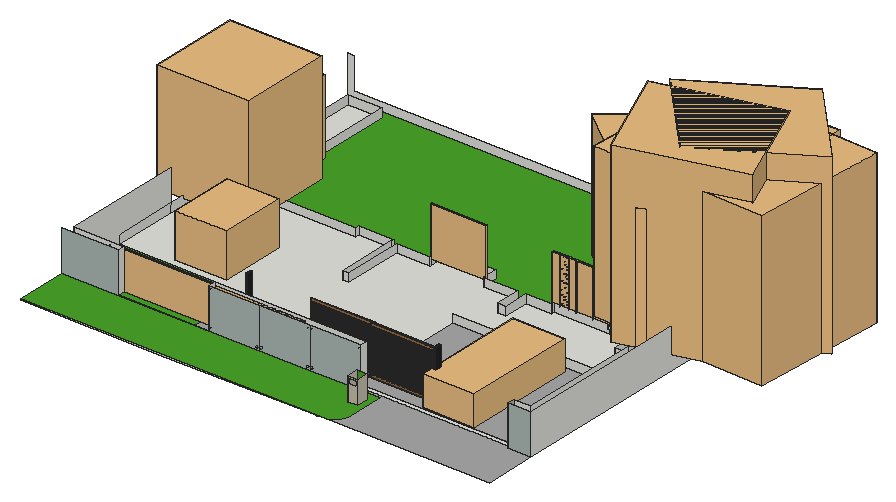
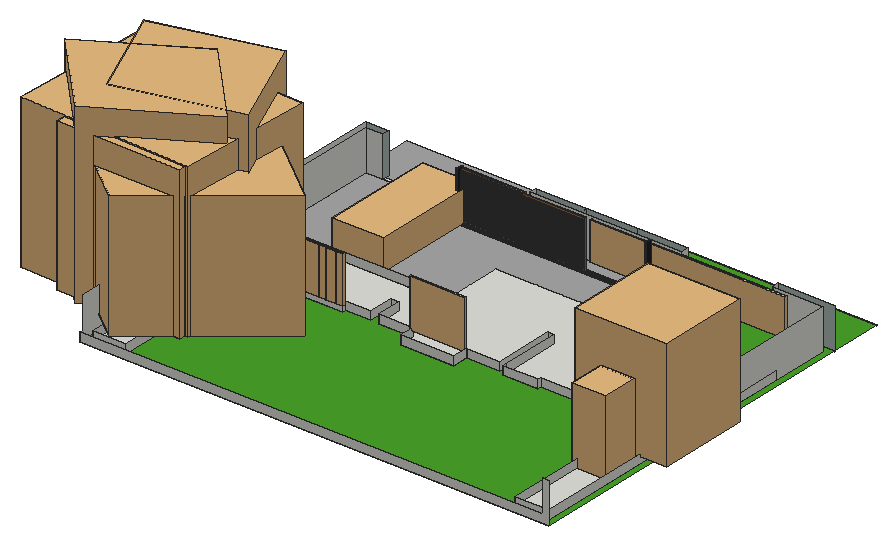
# SketchUp Ruby script. Lengths in inches.
U = 1.inch
M = Sketchup.active_model
def pt(a) = Geom::Point3d.new(a.map { |v| v * U })
def face(e, loops, mat)
  f = e.add_face(loops[0].map { |a| pt(a) })
  loops[1..].each { |l| e.add_face(l.map { |a| pt(a) }).erase! }
  f.material = f.back_material = mat if mat
  f
end
# faces: each face lists its corners as indices into pts; further lists are holes
def faces(e, pts, list, mat = nil) = list.each { |f| face(e, (f[0].is_a?(Array) ? f : [f]).map { |l| l.map { |i| pts[i] } }, mat) }
# xy, xz, yz: faces in a plane at the given z, y or x. An outline is a flat list of corners, or four numbers for a rectangle; further outlines are holes
def ring(l) = l.size == 4 ? [[l[0], l[1]], [l[2], l[1]], [l[2], l[3]], [l[0], l[3]]] : l.each_slice(2).to_a
def flat(e, list, mat, &to3) = list.each { |f| face(e, (f[0].is_a?(Array) ? f : [f]).map { |l| ring(l).map { |u, v| to3.(u, v) } }, mat) }
def xy(e, z, list, mat = nil) = flat(e, list, mat) { |x, y| [x, y, z] }
def xz(e, y, list, mat = nil) = flat(e, list, mat) { |x, z| [x, y, z] }
def yz(e, x, list, mat = nil) = flat(e, list, mat) { |y, z| [x, y, z] }
def lines(e, pts, list) = list.each { |a, b| e.add_line(pt(pts[a]), pt(pts[b])) }
# prism: a flat outline (further loops are holes) pulled along v
def prism(e, loops, v, mat = nil)
  f = face(e, loops, mat); d = Geom::Vector3d.new(v.map { |x| x * U })
  f.pushpull(f.normal.samedirection?(d) ? d.length : -d.length)
end
def box(e, o, s, mat = nil) = prism(e, [[o, [o[0] + s[0], o[1], o[2]], [o[0] + s[0], o[1] + s[1], o[2]], [o[0], o[1] + s[1], o[2]]]], [0, 0, s[2]], mat)
def at(x, y, z, deg = 0) = Geom::Transformation.translation(pt([x, y, z])) * Geom::Transformation.rotation(ORIGIN, Z_AXIS, deg.degrees)
def axes(o, x, y, z) = Geom::Transformation.new([*x, 0, *y, 0, *z, 0, *pt(o).to_a, 1])
def part(name) = M.definitions.add(name)
# library, detail: a bought-in or finely detailed component or shape, given as its bounding box
def library(name, o, s) = part(name).tap { |d| box(d.entities, o, s) }
def detail(e, o, s) = box(e.add_group.entities, o, s)
def put(e, d, t, mat = nil) = e.add_instance(d, t).tap { |i| i.material = mat if mat }
def group(e, t, mat = nil) = e.add_group.tap { |g| g.transformation = t; g.material = mat if mat }.entities
root = M.entities
M.materials.add("Material~3").color = [123, 113, 102]
M.materials.add("[0116_Lavender]").color = [73, 163, 41]
M.materials.add("[0132_LightGray]").color = [169, 169, 169]
M.materials.add("[0136_Charcoal]").color = [35, 35, 35]
M.materials.add("[Slate]").color = [172, 186, 182]
M.materials.add("[Tile Canvas]").color = [199, 192, 173]
M.materials.add("[Tile Grey]").color = [168, 168, 168]
M.materials.add("[Wood Floor Light]").color = [204, 176, 127]
M.materials.add("[Wood Floor]").color = [155, 105, 61]
c1 = library("Floor plant",[-5.56,-16.3125,0.81],[76.88,76.71,92.33])
c2 = library("Potted broadleaf plant",[-29.7,0,-10.87],[31.67,38.52,72.45])
c3 = library("Sem+nome (1)",[20.77,3.52,-2.22],[96.42,122.82,82.56])
c4 = library("Sliding Gate",[0,0,0],[194.88,4.13,70.58])
c5 = part("Group\#106")
box(c5.entities,[0,0,0],[3.9375,10.43,92.32])
c6 = library("3 door",[0,0,0],[74.8,3.9375,43.31])
c7 = part("Group\#107")
prism(c7.entities,[[[357.51,0,0.79],[357.51,0,-1.18],[357.51,10.43,-1.18],[357.51,10.43,0.79],[357.51,10.12,0.79],[357.51,10.12,0.39],[357.51,7.09,0.39],[357.51,7.09,0.79],[357.51,6.73,0.79],[357.51,6.73,0.39],[357.51,3.7,0.39],[357.51,3.7,0.79],[357.51,3.35,0.79],[357.51,3.35,0.39],[357.51,0.31,0.39],[357.51,0.31,0.79]]],[-357.51,0,0])
c8 = part("Group\#98")
box(c8.entities,[0,0,0],[1.57,1.97,82.68])
c9 = part("Group\#108")
g1 = group(c9.entities,at(0,0,0),"[Wood Floor]")
put(g1,c8,at(43.7,15.53,3.9375))
put(g1,c8,at(68.9,15.53,3.9375))
put(g1,c8,at(109.84,15.53,3.9375))
put(g1,c8,at(103.54,15.53,3.9375))
put(g1,c8,at(56.3,15.53,3.9375))
put(g1,c8,at(78.35,15.53,3.9375))
put(g1,c8,at(72.05,15.53,3.9375))
put(g1,c8,at(31.1,15.53,3.9375))
put(g1,c8,at(87.8,15.53,3.9375))
put(g1,c8,at(46.85,15.53,3.9375))
put(g1,c8,at(59.45,15.53,3.9375))
g2 = group(g1,at(12.2,15.53,3.9375))
box(g2,[0,0,0],[1.57,1.97,82.68])
put(g1,c8,at(50,15.53,3.9375))
put(g1,c8,at(106.69,15.53,3.9375))
put(g1,c8,at(34.25,15.53,3.9375))
put(g1,c8,at(81.5,15.53,3.9375))
put(g1,c8,at(53.15,15.53,3.9375))
put(g1,c8,at(27.95,15.53,3.9375))
put(g1,c8,at(65.75,15.53,3.9375))
put(g1,c8,at(18.5,15.53,3.9375))
put(g1,c8,at(40.55,15.53,3.9375))
put(g1,c8,at(75.2,15.53,3.9375))
put(g1,c8,at(21.65,15.53,3.9375))
put(g1,c8,at(62.6,15.53,3.9375))
put(g1,c8,at(84.65,15.53,3.9375))
put(g1,c8,at(100.39,15.53,3.9375))
put(g1,c8,at(112.99,15.53,3.9375))
put(g1,c8,at(24.8,15.53,3.9375))
put(g1,c8,at(37.4,15.53,3.9375))
put(g1,c8,at(97.24,15.53,3.9375))
put(g1,c8,at(2.76,15.53,3.9375))
g3 = group(g1,at(5.91,15.53,3.9375))
box(g3,[0,0,0],[1.57,1.97,82.68])
put(g1,c8,at(94.09,15.53,3.9375))
put(g1,c8,at(15.35,15.53,3.9375))
put(g1,c8,at(9.06,15.53,3.9375))
put(g1,c8,at(90.94,15.53,3.9375))
g4 = group(c9.entities,at(0,14.54,0))
xy(g4,0,[[0,0,118.11,2.95]],"[Wood Floor]")
xy(g4,3.9375,[[2.76,0,115.35,2.95]],"[Wood Floor]")
xy(g4,30.51,[[2.76,0,115.35,0.98]],"[Wood Floor]")
xy(g4,31.5,[[2.76,0,115.35,0.98]],"[Wood Floor]")
xy(g4,42.19,[[1.12,0,1.91,0.79]],"[Wood Floor]")
xy(g4,42.49,[[116.24,2.17,117.03,2.95]],"[Wood Floor]")
xy(g4,46.92,[[1.12,0,1.91,0.79]],"[Wood Floor]")
xy(g4,47.22,[[116.24,2.17,117.03,2.95]],"[Wood Floor]")
xy(g4,58.07,[[2.76,0,115.35,0.98]],"[Wood Floor Light]")
xy(g4,59.06,[[2.76,0,115.35,0.98]],"[Wood Floor]")
xy(g4,86.61,[[2.76,0,115.35,2.95]],"[Wood Floor]")
xy(g4,90.55,[[0,0,118.11,2.95]],"[Wood Floor]")
xz(g4,0,[[2.76,30.51,115.35,31.5],[2.76,58.07,115.35,59.06]],"[Wood Floor Light]")
xz(g4,0,[[[0,0,118.11,90.55],[2.76,3.9375,115.35,86.61],[1.12,42.19,1.91,46.92]]],"[Wood Floor]")
xz(g4,0.79,[[1.12,42.19,1.91,46.92]],"[Wood Floor]")
xz(g4,0.98,[[2.76,30.51,115.35,31.5],[2.76,58.07,115.35,59.06]],"[Wood Floor]")
xz(g4,2.17,[[116.24,42.49,117.03,47.22]],"[Wood Floor]")
xz(g4,2.95,[[[0,0,118.11,90.55],[2.76,3.9375,115.35,86.61],[116.24,42.49,117.03,47.22]]],"[Wood Floor]")
yz(g4,0,[[0,0,2.95,90.55]],"[Wood Floor]")
yz(g4,1.12,[[0,42.19,0.79,46.92]],"[Wood Floor]")
yz(g4,1.91,[[0,42.19,0.79,46.92]],"[Wood Floor]")
yz(g4,2.76,[[0,3.9375,2.95,3.9375,2.95,86.61,0,86.61,0,59.06,0.98,59.06,0.98,58.07,0,58.07,0,31.5,0.98,31.5,0.98,30.51,0,30.51],[0,30.51,0.98,31.5],[0,58.07,0.98,59.06]],"[Wood Floor]")
yz(g4,115.35,[[0,3.9375,0,30.51,0.98,30.51,0.98,31.5,0,31.5,0,58.07,0.98,58.07,0.98,59.06,0,59.06,0,86.61,2.95,86.61,2.95,3.9375],[0,30.51,0.98,31.5],[0,58.07,0.98,59.06]],"[Wood Floor]")
yz(g4,116.24,[[2.17,42.49,2.95,47.22]],"[Wood Floor]")
yz(g4,117.03,[[2.17,42.49,2.95,47.22]],"[Wood Floor]")
yz(g4,118.11,[[0,0,2.95,90.55]],"[Wood Floor]")
p = [[5.91,2.95,86.61],[5.91,2.95,3.9375]]
lines(g4,p,[[0,1]])
c10 = part("Group\#103")
put(c10.entities,c8,at(43.7,15.53,3.9375))
put(c10.entities,c8,at(68.9,15.53,3.9375))
put(c10.entities,c8,at(109.84,15.53,3.9375))
put(c10.entities,c8,at(103.54,15.53,3.9375))
put(c10.entities,c8,at(56.3,15.53,3.9375))
put(c10.entities,c8,at(78.35,15.53,3.9375))
put(c10.entities,c8,at(72.05,15.53,3.9375))
put(c10.entities,c8,at(31.1,15.53,3.9375))
put(c10.entities,c8,at(87.8,15.53,3.9375))
put(c10.entities,c8,at(46.85,15.53,3.9375))
put(c10.entities,c8,at(59.45,15.53,3.9375))
put(c10.entities,c8,at(12.2,15.53,3.9375))
put(c10.entities,c8,at(50,15.53,3.9375))
put(c10.entities,c8,at(106.69,15.53,3.9375))
put(c10.entities,c8,at(34.25,15.53,3.9375))
put(c10.entities,c8,at(81.5,15.53,3.9375))
put(c10.entities,c8,at(53.15,15.53,3.9375))
put(c10.entities,c8,at(27.95,15.53,3.9375))
put(c10.entities,c8,at(65.75,15.53,3.9375))
put(c10.entities,c8,at(18.5,15.53,3.9375))
put(c10.entities,c8,at(40.55,15.53,3.9375))
put(c10.entities,c8,at(75.2,15.53,3.9375))
put(c10.entities,c8,at(21.65,15.53,3.9375))
put(c10.entities,c8,at(62.6,15.53,3.9375))
put(c10.entities,c8,at(84.65,15.53,3.9375))
put(c10.entities,c8,at(100.39,15.53,3.9375))
put(c10.entities,c8,at(112.99,15.53,3.9375))
put(c10.entities,c8,at(24.8,15.53,3.9375))
put(c10.entities,c8,at(37.4,15.53,3.9375))
put(c10.entities,c8,at(97.24,15.53,3.9375))
put(c10.entities,c8,at(2.76,15.53,3.9375))
put(c10.entities,c8,at(5.91,15.53,3.9375))
put(c10.entities,c8,at(94.09,15.53,3.9375))
put(c10.entities,c8,at(15.35,15.53,3.9375))
put(c10.entities,c8,at(9.06,15.53,3.9375))
put(c10.entities,c8,at(90.94,15.53,3.9375))
c11 = part("Group\#104")
put(c11.entities,c10,at(0,0,0),"[Wood Floor]")
g5 = group(c11.entities,at(0,14.54,0))
xy(g5,0,[[0,0,118.11,2.95]],"[Wood Floor]")
xy(g5,3.9375,[[2.76,0,115.35,2.95]],"[Wood Floor]")
xy(g5,30.51,[[2.76,0,115.35,0.98]],"[Wood Floor]")
xy(g5,31.5,[[2.76,0,115.35,0.98]],"[Wood Floor]")
xy(g5,42.07,[[116.14,2.17,116.92,2.95]],"[Wood Floor]")
xy(g5,42.125,[[1.06,0,1.84,0.79]],"[Wood Floor]")
xy(g5,46.8,[[116.14,2.17,116.92,2.95]],"[Wood Floor]")
xy(g5,46.85,[[1.06,0,1.84,0.79]],"[Wood Floor]")
xy(g5,58.07,[[2.76,0,115.35,0.98]],"[Wood Floor Light]")
xy(g5,59.06,[[2.76,0,115.35,0.98]],"[Wood Floor]")
xy(g5,86.61,[[2.76,0,115.35,2.95]],"[Wood Floor]")
xy(g5,90.55,[[0,0,118.11,2.95]],"[Wood Floor]")
xz(g5,0,[[2.76,30.51,115.35,31.5],[2.76,58.07,115.35,59.06]],"[Wood Floor Light]")
xz(g5,0,[[[0,0,118.11,90.55],[2.76,3.9375,115.35,86.61],[1.06,42.125,1.84,46.85]]],"[Wood Floor]")
xz(g5,0.79,[[1.06,42.125,1.84,46.85]],"[Wood Floor]")
xz(g5,0.98,[[2.76,30.51,115.35,31.5],[2.76,58.07,115.35,59.06]],"[Wood Floor]")
xz(g5,2.17,[[116.14,42.07,116.92,46.8]],"[Wood Floor]")
xz(g5,2.95,[[[0,0,118.11,90.55],[2.76,3.9375,115.35,86.61],[116.14,42.07,116.92,46.8]]],"[Wood Floor]")
yz(g5,0,[[0,0,2.95,90.55]],"[Wood Floor]")
yz(g5,1.06,[[0,42.125,0.79,46.85]],"[Wood Floor]")
yz(g5,1.84,[[0,42.125,0.79,46.85]],"[Wood Floor]")
yz(g5,2.76,[[0,3.9375,2.95,3.9375,2.95,86.61,0,86.61,0,59.06,0.98,59.06,0.98,58.07,0,58.07,0,31.5,0.98,31.5,0.98,30.51,0,30.51],[0,30.51,0.98,31.5],[0,58.07,0.98,59.06]],"[Wood Floor]")
yz(g5,115.35,[[0,3.9375,0,30.51,0.98,30.51,0.98,31.5,0,31.5,0,58.07,0.98,58.07,0.98,59.06,0,59.06,0,86.61,2.95,86.61,2.95,3.9375],[0,30.51,0.98,31.5],[0,58.07,0.98,59.06]],"[Wood Floor]")
yz(g5,116.14,[[2.17,42.07,2.95,46.8]],"[Wood Floor]")
yz(g5,116.92,[[2.17,42.07,2.95,46.8]],"[Wood Floor]")
yz(g5,118.11,[[0,0,2.95,90.55]],"[Wood Floor]")
p = [[5.91,2.95,86.61],[5.91,2.95,3.9375]]
lines(g5,p,[[0,1]])
c12 = library("3DGeom~4_Defintion",[362.52,-15.59,12.6],[288.85,70.11,1000])
c13 = library("BMW 8 Series M850i 2019",[-14.25,0.77,-0.16],[87.38,190.63,50.87])
c14 = library("Group\#65",[-33.32,-34.9375,32.67],[162.87,159.66,128.34])
c15 = library("Group\#81",[-10.45,-6.67,0],[121.7,116.61,164.95])
c16 = library("Group\#82",[-10.45,-6.67,0],[121.7,116.61,164.95])
c17 = library("Group\#69",[-10.45,-6.67,0],[121.7,116.61,164.95])
c18 = library("Group\#83",[-33.32,-34.9375,32.67],[162.87,159.66,128.34])
c19 = library("Group\#64",[-33.32,-34.9375,81.35],[162.87,159.66,79.66])
c20 = library("Group\#80",[-33.32,-34.9375,77.91],[162.87,159.66,83.1])
c21 = part("Palem Elek")
put(c21.entities,c14,axes([92.2,20.3,-29.73],[0.70711,0.70711,0],[-0.70711,0.70711,0],[0,0,0.91208]))
put(c21.entities,c15,axes([60.27,20.78,0],[1,0,0],[0,1,0],[0,0,0.85762]))
put(c21.entities,c16,at(25.45,60.83,0,-53.5))
put(c21.entities,c17,at(84.4375,135.48,0,-161.4))
put(c21.entities,c18,axes([38.54,105.7,-36.19],[-0.04013,-0.99919,0],[0.99919,-0.04013,0],[0,0,1.11001]))
put(c21.entities,c19,axes([57.15,96.51,-54.45],[-0.02003,-0.49872,0.02965],[0.4996,-0.02007,0],[0.00123,0.03065,0.51628]))
put(c21.entities,c20,axes([74.94,50.39,-54.06],[0.40095,0.29715,0.03075],[-0.29654,0.38966,0.10114],[0.04012,-0.11026,0.54246]))
c22 = part("palem elek\#1")
put(c22.entities,c21,at(-81.14,-74.56,-0.83))
c23 = part("Coqueiro")
put(c23.entities,c22,axes([83.17,89.39,9.5625],[0,1.1016,0],[-1.377,0,0],[0,0,1.39284]))
xy(root,-10.51,[[1716.62,498.28,1993.42,505.1],[[1168.49,611.53,1168.49,1146.63,1232.12,1146.63,1232.12,732.28,1243.06,732.28,1243.06,845.35,1425.1,845.35,1425.1,851.0625,1490.48,851.0625,1490.48,732.28,1501.42,732.28,1501.42,845.35,1564.1,845.35,1564.1,874.25,1664.38,874.25,1664.38,845.35,1728.67,845.35,1728.67,798.41,1744,798.41,1744,845.35,1791.45,845.35,1791.45,851.0625,1960.87,851.0625,1960.87,1146.63,2024.12,1146.63,2024.12,732.28,1696.41,732.28,1696.41,611.53],[1945.54,801.78,1960.87,845.35]]])
xy(root,-10.51,[[[1156.87,393.78,1727.12,393.78,1730.14,394.71,1733.08,395.9,1735.89,397.35,1738.57,399.04,1741.08,400.97,1743.42,403.1,1745.56,405.44,1747.48,407.96,1749.17,410.63,1750.62,413.45,1751.8125,416.38,1752.74,419.41,1752.74,491.47,1716.62,491.47,1716.62,505.1,1431.76,505.1,1431.76,491.47,1262.76,491.47,1262.76,505.1,1168.49,505.1,1168.49,1146.63,1232.12,1146.63,1232.12,732.28,1243.06,732.28,1243.06,845.35,1425.1,845.35,1425.1,851.0625,1490.48,851.0625,1490.48,732.28,1501.42,732.28,1501.42,845.35,1564.1,845.35,1564.1,874.25,1664.38,874.25,1664.38,845.35,1728.67,845.35,1728.67,798.41,1744,798.41,1744,845.35,1791.45,845.35,1791.45,851.0625,1960.87,851.0625,1960.87,1146.63,2024.12,1146.63,2024.12,505.1,1993.42,505.1,1993.42,491.47,2036.12,491.47,2036.12,1160.85,1156.87,1160.85],[1722.63,453.42,1741.07,475.99]],[1262.76,491.47,1406.2,491.47,1411.4,611.53,1168.49,611.53,1168.49,505.1,1262.76,505.1]],"[0116_Lavender]")
xy(root,-10.51,[[1727.12,393.78,2036.12,393.78,2036.12,491.47,1993.42,491.47,1993.42,498.28,1716.62,498.28,1716.62,491.47,1752.74,491.47,1752.74,419.41,1751.8125,416.38,1750.62,413.45,1749.17,410.63,1747.48,407.96,1745.56,405.44,1743.42,403.1,1741.08,400.97,1738.57,399.04,1735.89,397.35,1733.08,395.9,1730.14,394.71],[1406.2,491.47,1431.76,491.47,1431.76,505.1,2024.12,505.1,2024.12,732.28,1696.41,732.28,1696.41,611.53,1411.4,611.53]],"[Tile Grey]")
xz(root,393.78,[[1156.87,-12.6875,1431.76,-12.6875,1716.62,-10.51,1156.87,-10.51]])
xz(root,453.42,[[[1722.63,-10.51,1741.07,32.74],[1724.98,19.53,1739.11,29.34]]],"[Tile Canvas]")
xz(root,475.99,[[1722.63,-10.51,1741.07,32.74]],"[0116_Lavender]")
xz(root,491.47,[[1262.76,-12.6875,1431.76,-10.51]])
xz(root,491.47,[[1522.98,-7.89,1523.46,-7.82,1523.92,-7.63,1524.3,-7.34,1524.6,-6.95,1524.79,-6.5,1524.85,-6.01,1524.79,-5.52,1524.6,-5.07,1524.3,-4.68,1523.92,-4.39,1523.46,-4.2,1522.98,-4.14,1522.49,-4.2,1522.04,-4.39,1521.65,-4.68,1521.36,-5.07,1521.17,-5.52,1521.1,-6.01,1521.17,-6.5,1521.36,-6.95,1521.65,-7.34,1522.04,-7.63,1522.49,-7.82],[1617.93,-7.89,1618.41,-7.82,1618.87,-7.63,1619.26,-7.34,1619.55,-6.95,1619.74,-6.5,1619.8,-6.01,1619.74,-5.52,1619.55,-5.07,1619.26,-4.68,1618.87,-4.39,1618.41,-4.2,1617.93,-4.14,1617.44,-4.2,1616.99,-4.39,1616.6,-4.68,1616.31,-5.07,1616.12,-5.52,1616.05,-6.01,1616.12,-6.5,1616.31,-6.95,1616.6,-7.34,1616.99,-7.63,1617.44,-7.82],[1712.88,-7.89,1713.37,-7.82,1713.82,-7.63,1714.21,-7.34,1714.5,-6.95,1714.69,-6.5,1714.76,-6.01,1714.69,-5.52,1714.5,-5.07,1714.21,-4.68,1713.82,-4.39,1713.37,-4.2,1712.88,-4.14,1712.4,-4.2,1711.94,-4.39,1711.55,-4.68,1711.26,-5.07,1711.07,-5.52,1711.01,-6.01,1711.07,-6.5,1711.26,-6.95,1711.55,-7.34,1711.94,-7.63,1712.4,-7.82],[1435.25,-6.41,1435.73,-6.4,1436.2,-6.26,1436.62,-6.01,1436.96,-5.66,1437.19,-5.23,1437.31,-4.75,1437.3,-4.26,1437.16,-3.79,1436.9,-3.375,1436.55,-3.04,1436.12,-2.8,1435.65,-2.6875,1435.16,-2.7,1434.6875,-2.84,1434.27,-3.09,1433.93,-3.45,1433.7,-3.875,1433.58,-4.35,1433.59,-4.84,1433.73,-5.31,1433.99,-5.73,1434.34,-6.07,1434.77,-6.3],[1530.2,-6.41,1530.6875,-6.4,1531.16,-6.26,1531.57,-6.01,1531.91,-5.66,1532.15,-5.23,1532.26,-4.75,1532.25,-4.26,1532.11,-3.79,1531.86,-3.375,1531.5,-3.04,1531.07,-2.8,1530.6,-2.6875,1530.11,-2.7,1529.64,-2.84,1529.22,-3.09,1528.88,-3.45,1528.65,-3.875,1528.53,-4.35,1528.54,-4.84,1528.68,-5.31,1528.9375,-5.73,1529.29,-6.07,1529.72,-6.3],
  [1625.15,-6.41,1625.64,-6.4,1626.11,-6.26,1626.52,-6.01,1626.86,-5.66,1627.1,-5.23,1627.21,-4.75,1627.2,-4.26,1627.0625,-3.79,1626.81,-3.375,1626.45,-3.04,1626.02,-2.8,1625.55,-2.6875,1625.06,-2.7,1624.59,-2.84,1624.17,-3.09,1623.83,-3.45,1623.6,-3.875,1623.48,-4.35,1623.49,-4.84,1623.63,-5.31,1623.89,-5.73,1624.24,-6.07,1624.67,-6.3]],"[0132_LightGray]")
xz(root,491.47,[[1156.87,-12.6875,1262.76,65.1875],[[1431.76,-12.6875,1716.62,-10.51,1716.62,65.1875,1431.76,65.1875],[1522.98,-7.89,1522.49,-7.82,1522.04,-7.63,1521.65,-7.34,1521.36,-6.95,1521.17,-6.5,1521.1,-6.01,1521.17,-5.52,1521.36,-5.07,1521.65,-4.68,1522.04,-4.39,1522.49,-4.2,1522.98,-4.14,1523.46,-4.2,1523.92,-4.39,1524.3,-4.68,1524.6,-5.07,1524.79,-5.52,1524.85,-6.01,1524.79,-6.5,1524.6,-6.95,1524.3,-7.34,1523.92,-7.63,1523.46,-7.82],[1617.93,-7.89,1617.44,-7.82,1616.99,-7.63,1616.6,-7.34,1616.31,-6.95,1616.12,-6.5,1616.05,-6.01,1616.12,-5.52,1616.31,-5.07,1616.6,-4.68,1616.99,-4.39,1617.44,-4.2,1617.93,-4.14,1618.41,-4.2,1618.87,-4.39,1619.26,-4.68,1619.55,-5.07,1619.74,-5.52,1619.8,-6.01,1619.74,-6.5,1619.55,-6.95,1619.26,-7.34,1618.87,-7.63,1618.41,-7.82],[1522.98,57.74,1522.49,57.8,1522.04,57.99,1521.65,58.29,1521.36,58.68,1521.17,59.13,1521.1,59.61,1521.17,60.1,1521.36,60.55,1521.65,60.94,1522.04,61.24,1522.49,61.43,1522.98,61.49,1523.46,61.43,1523.92,61.24,1524.3,60.94,1524.6,60.55,1524.79,60.1,1524.85,59.61,1524.79,59.13,1524.6,58.68,1524.3,58.29,1523.92,57.99,1523.46,57.8],[1617.93,57.74,1617.44,57.8,1616.99,57.99,1616.6,58.29,1616.31,58.68,1616.12,59.13,1616.05,59.61,1616.12,60.1,1616.31,60.55,1616.6,60.94,1616.99,61.24,1617.44,61.43,1617.93,61.49,1618.41,61.43,1618.87,61.24,1619.26,60.94,1619.55,60.55,1619.74,60.1,1619.8,59.61,1619.74,59.13,1619.55,58.68,1619.26,58.29,1618.87,57.99,1618.41,57.8],[1712.88,-7.89,1712.4,-7.82,1711.94,-7.63,1711.55,-7.34,1711.26,-6.95,1711.07,-6.5,1711.01,-6.01,1711.07,-5.52,1711.26,-5.07,1711.55,-4.68,1711.94,-4.39,1712.4,-4.2,1712.88,-4.14,1713.37,-4.2,1713.82,-4.39,1714.21,-4.68,1714.5,-5.07,1714.69,-5.52,1714.76,-6.01,1714.69,-6.5,1714.5,-6.95,1714.21,-7.34,1713.82,-7.63,1713.37,-7.82],[1712.88,57.74,1712.4,57.8,1711.94,57.99,1711.55,58.29,1711.26,58.68,1711.07,59.13,1711.01,59.61,1711.07,60.1,1711.26,60.55,1711.55,60.94,1711.94,61.24,1712.4,61.43,1712.88,61.49,1713.37,61.43,1713.82,61.24,1714.21,60.94,1714.5,60.55,1714.69,60.1,1714.76,59.61,1714.69,59.13,1714.5,58.68,1714.21,58.29,1713.82,57.99,1713.37,57.8],[1530.2,59.21,1529.72,59.33,1529.29,59.56,1528.9375,59.9,1528.68,60.32,1528.54,60.78,1528.53,61.27,1528.65,61.75,1528.88,62.18,1529.22,62.53,1529.64,62.79,1530.11,62.93,1530.6,62.9375,1531.07,62.82,1531.5,62.59,1531.86,62.25,1532.11,61.83,1532.25,61.36,1532.26,60.875,1532.15,60.4,1531.91,59.97,1531.57,59.61,1531.16,59.36,1530.6875,59.22],[1625.15,59.21,1624.67,59.33,1624.24,59.56,1623.89,59.9,1623.63,60.32,1623.49,60.78,1623.48,61.27,1623.6,61.75,1623.83,62.18,1624.17,62.53,1624.59,62.79,1625.06,62.93,1625.55,62.9375,1626.02,62.82,1626.45,62.59,1626.81,62.25,1627.0625,61.83,1627.2,61.36,1627.21,60.875,1627.1,60.4,1626.86,59.97,1626.52,59.61,1626.11,59.36,1625.64,59.22],[1435.25,-6.41,1434.77,-6.3,1434.34,-6.07,1433.99,-5.73,1433.73,-5.31,1433.59,-4.84,1433.58,-4.35,1433.7,-3.875,1433.93,-3.45,1434.27,-3.09,1434.6875,-2.84,1435.16,-2.7,1435.65,-2.6875,1436.12,-2.8,1436.55,-3.04,1436.9,-3.375,1437.16,-3.79,1437.3,-4.26,1437.31,-4.75,1437.19,-5.23,1436.96,-5.66,1436.62,-6.01,1436.2,-6.26,1435.73,-6.4],[1530.2,-6.41,1529.72,-6.3,1529.29,-6.07,1528.9375,-5.73,1528.68,-5.31,1528.54,-4.84,1528.53,-4.35,1528.65,-3.875,1528.88,-3.45,1529.22,-3.09,1529.64,-2.84,1530.11,-2.7,1530.6,-2.6875,1531.07,-2.8,1531.5,-3.04,1531.86,-3.375,1532.11,-3.79,1532.25,-4.26,1532.26,-4.75,1532.15,-5.23,1531.91,-5.66,1531.57,-6.01,1531.16,-6.26,1530.6875,-6.4],[1625.15,-6.41,1624.67,-6.3,1624.24,-6.07,1623.89,-5.73,1623.63,-5.31,1623.49,-4.84,1623.48,-4.35,1623.6,-3.875,1623.83,-3.45,1624.17,-3.09,1624.59,-2.84,1625.06,-2.7,1625.55,-2.6875,1626.02,-2.8,1626.45,-3.04,1626.81,-3.375,1627.0625,-3.79,1627.2,-4.26,1627.21,-4.75,1627.1,-5.23,1626.86,-5.66,1626.52,-6.01,1626.11,-6.26,1625.64,-6.4],[1435.25,59.21,1434.77,59.33,1434.34,59.56,1433.99,59.9,1433.73,60.32,1433.59,60.78,1433.58,61.27,1433.7,61.75,1433.93,62.18,1434.27,62.53,1434.6875,62.79,1435.16,62.93,1435.65,62.9375,1436.12,62.82,1436.55,62.59,1436.9,62.25,1437.16,61.83,1437.3,61.36,1437.31,60.875,1437.19,60.4,1436.96,59.97,1436.62,59.61,1436.2,59.36,1435.73,59.22]],[1993.42,-10.51,2036.12,65.1875]],"[Slate]")
xz(root,505.1,[[1168.49,-10.51,1262.76,65.1875],[1431.76,-10.51,1716.62,65.1875],[1993.42,-10.51,2024.12,65.1875]])
xz(root,732.28,[[1232.12,-10.51,1243.06,5.1875],[1490.48,-10.51,1501.42,5.1875],[1696.41,-10.51,2024.12,5.1875]])
xz(root,798.41,[[1728.67,-10.51,1744,5.1875]])
xz(root,801.78,[[1945.54,-10.51,1960.87,5.1875]])
xz(root,845.35,[[1243.06,-10.51,1425.1,5.1875],[1501.42,-10.51,1564.1,5.1875],[1664.38,-10.51,1728.67,5.1875],[1744,-10.51,1791.45,5.1875],[1945.54,-10.51,1960.87,5.1875],
  [1896.07,-0.125,1945.54,5.1875]])
xz(root,851.0625,[[1425.1,-10.51,1490.48,5.1875],[1791.45,-10.51,1896.07,5.1875],[1896.07,-10.51,1955.15,5.1875],[1955.15,-10.51,1960.87,5.1875]])
xz(root,874.25,[[1564.1,-10.51,1664.38,5.1875]])
xz(root,1146.63,[[1168.49,-10.51,1232.12,5.1875],[1960.87,-10.51,2024.12,5.1875]])
xz(root,1160.85,[[1156.87,-10.51,1156.87,65.1875,1168.49,65.1875,1168.49,5.1875,2036.12,5.1875,2036.12,-10.51]])
yz(root,1168.49,[[505.1,-10.51,611.53,-10.51,611.53,5.1875,732.28,5.1875,732.28,65.1875,505.1,65.1875],[611.53,-10.51,732.28,5.1875],[732.28,-10.51,1146.63,5.1875]])
yz(root,1232.12,[[732.28,-10.51,1146.63,5.1875]])
yz(root,1243.06,[[732.28,-10.51,845.35,5.1875]])
yz(root,1262.76,[[491.47,-10.51,505.1,65.1875]])
yz(root,1425.1,[[845.35,-10.51,851.0625,5.1875]])
yz(root,1431.76,[[491.47,-10.51,505.1,65.1875]])
yz(root,1490.48,[[732.28,-10.51,846.1,5.1875],[846.1,-10.51,851.0625,5.1875]])
yz(root,1501.42,[[732.28,-10.51,845.35,5.1875]])
yz(root,1564.1,[[845.35,-10.51,846.1,5.1875],[846.1,-10.51,874.25,5.1875]])
yz(root,1664.38,[[845.35,-10.51,846.1,5.1875],[846.1,-10.51,874.25,5.1875]])
yz(root,1716.62,[[491.47,-10.51,505.1,65.1875]])
yz(root,1722.63,[[453.42,-10.51,475.99,32.74]],"[Tile Canvas]")
yz(root,1728.67,[[798.41,-10.51,845.35,5.1875]])
yz(root,1741.07,[[453.42,-10.51,475.99,32.74]],"[Tile Canvas]")
yz(root,1744,[[798.41,-10.51,845.35,5.1875]])
yz(root,1791.45,[[845.35,-10.51,846.1,5.1875],[846.1,-10.51,851.0625,5.1875]])
yz(root,1896.07,[[845.35,-0.125,851.0625,5.1875]])
yz(root,1945.54,[[801.78,-10.51,845.35,5.1875]])
yz(root,1960.87,[[801.78,-10.51,845.35,5.1875],[851.0625,-10.51,1146.63,5.1875]])
yz(root,1993.42,[[491.47,-10.51,505.1,65.1875]],"[Slate]")
yz(root,2024.12,[[505.1,-10.51,732.28,65.1875],[732.28,-10.51,1146.63,5.1875]])
yz(root,2036.12,[[491.47,-10.51,1160.85,-10.51,1160.85,5.1875,1155.13,5.1875,1155.13,65.1875,491.47,65.1875]])
p = [[1707.05,532.58,-10.51],[1705.91,532.58,-10.51],[1526.71,491.47,65.1875],[1526.71,491.47,-10.51],[1621.66,491.47,65.1875],[1621.66,491.47,-10.51]]
lines(root,p,[[0,1],[2,3],[4,5]])
put(root,c1,axes([1131.29,797.14,-1],[2.24,0,0],[0,2.24,0],[0,0,2.24]))
put(root,c2,axes([1237.75,858.27,6.22],[2,0,0],[0,2,0],[0,0,2]))
put(root,c2,axes([1237.75,924.09,6.22],[2,0,0],[0,2,0],[0,0,2]))
put(root,c3,at(1248.88,611.53,-0.125))
put(root,c4,axes([1235.32,505.1,-10.51],[1.88,0,0],[0,1,0],[0,0,1]))
put(root,c5,at(1469.29,530.57,-10.11),"[0136_Charcoal]")
put(root,c6,axes([1564.1,846.14,1.53],[1.37387,0,0],[0,0.86071,0],[0,0,2.11056]))
put(root,c7,at(1469.29,530.57,-10.51),"[0136_Charcoal]")
put(root,c9,at(1589.32,519.73,-10.11))
put(root,c11,at(1704.68,516.42,-9.72))
put(root,c12,axes([1747.75,854.26,0.98],[0.11056,0,0],[0,-0.05859,0],[0,0,0.08734]),"Material~3")
put(root,c12,axes([1761.79,854.26,0.98],[0.11056,0,0],[0,-0.05859,0],[0,0,0.08734]),"Material~3")
put(root,c5,at(1822.87,530.57,-10.11),"[0136_Charcoal]")
put(root,c12,axes([1792.37,854.26,0.98],[0.11056,0,0],[0,-0.05859,0],[0,0,0.08734]),"Material~3")
put(root,c13,axes([1900.1,720.81,-10.33],[-1.11,0,0],[0,-1.11,0],[0,0,1.11]))
put(root,c12,axes([1824.06,854.26,0.98],[0.11056,0,0],[0,-0.05859,0],[0,0,0.08734]),"Material~3")
put(root,c23,axes([1887.42,830.17,6.32],[1.44,0,0],[0,1.44,0],[0,0,1.44]))
